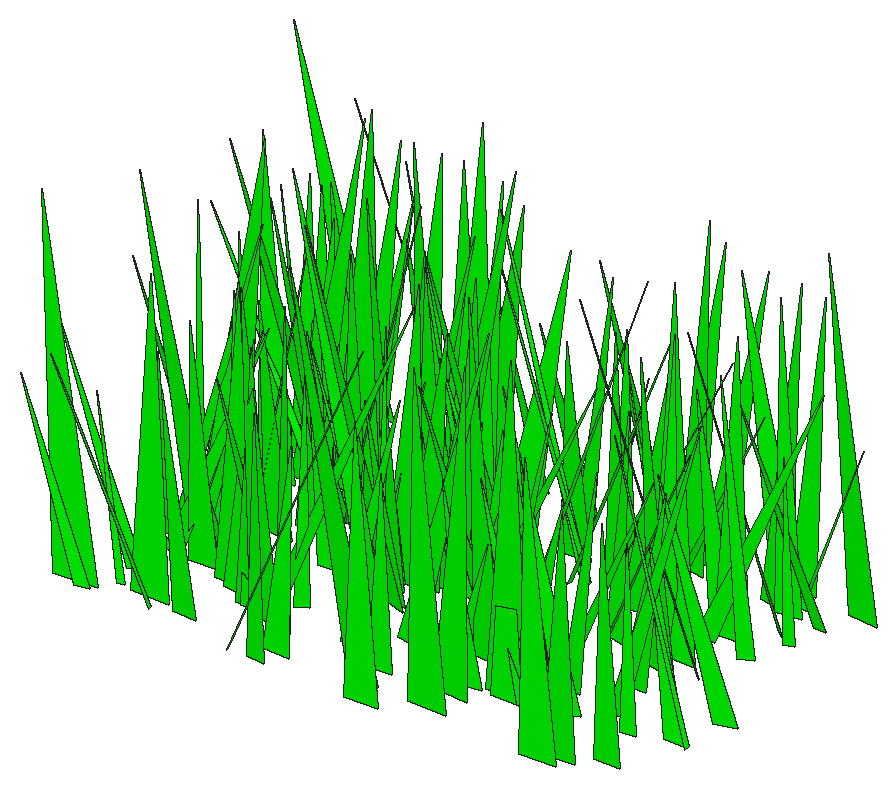
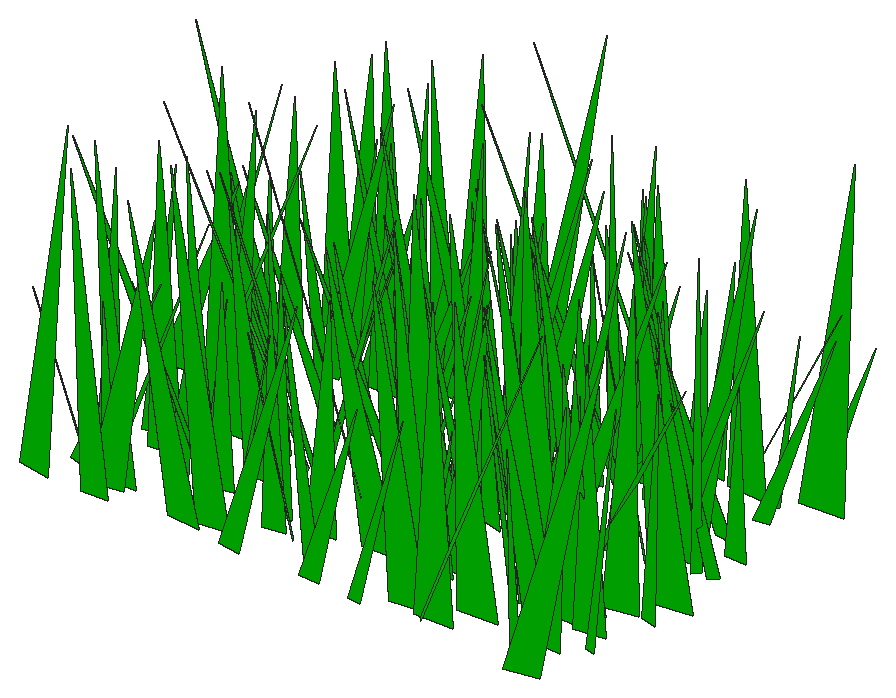
# SketchUp Ruby script. Lengths in inches.
U = 1.inch
M = Sketchup.active_model
def pt(a) = Geom::Point3d.new(a.map { |v| v * U })
def face(e, loops, mat)
  f = e.add_face(loops[0].map { |a| pt(a) })
  loops[1..].each { |l| e.add_face(l.map { |a| pt(a) }).erase! }
  f.material = f.back_material = mat if mat
  f
end
# faces: each face lists its corners as indices into pts; further lists are holes
def faces(e, pts, list, mat = nil) = list.each { |f| face(e, (f[0].is_a?(Array) ? f : [f]).map { |l| l.map { |i| pts[i] } }, mat) }
# xy, xz, yz: faces in a plane at the given z, y or x. An outline is a flat list of corners, or four numbers for a rectangle; further outlines are holes
def ring(l) = l.size == 4 ? [[l[0], l[1]], [l[2], l[1]], [l[2], l[3]], [l[0], l[3]]] : l.each_slice(2).to_a
def flat(e, list, mat, &to3) = list.each { |f| face(e, (f[0].is_a?(Array) ? f : [f]).map { |l| ring(l).map { |u, v| to3.(u, v) } }, mat) }
def xy(e, z, list, mat = nil) = flat(e, list, mat) { |x, y| [x, y, z] }
def xz(e, y, list, mat = nil) = flat(e, list, mat) { |x, z| [x, y, z] }
def yz(e, x, list, mat = nil) = flat(e, list, mat) { |y, z| [x, y, z] }
def lines(e, pts, list) = list.each { |a, b| e.add_line(pt(pts[a]), pt(pts[b])) }
# prism: a flat outline (further loops are holes) pulled along v
def prism(e, loops, v, mat = nil)
  f = face(e, loops, mat); d = Geom::Vector3d.new(v.map { |x| x * U })
  f.pushpull(f.normal.samedirection?(d) ? d.length : -d.length)
end
def box(e, o, s, mat = nil) = prism(e, [[o, [o[0] + s[0], o[1], o[2]], [o[0] + s[0], o[1] + s[1], o[2]], [o[0], o[1] + s[1], o[2]]]], [0, 0, s[2]], mat)
def at(x, y, z, deg = 0) = Geom::Transformation.translation(pt([x, y, z])) * Geom::Transformation.rotation(ORIGIN, Z_AXIS, deg.degrees)
def axes(o, x, y, z) = Geom::Transformation.new([*x, 0, *y, 0, *z, 0, *pt(o).to_a, 1])
def part(name) = M.definitions.add(name)
# library, detail: a bought-in or finely detailed component or shape, given as its bounding box
def library(name, o, s) = part(name).tap { |d| box(d.entities, o, s) }
def detail(e, o, s) = box(e.add_group.entities, o, s)
def put(e, d, t, mat = nil) = e.add_instance(d, t).tap { |i| i.material = mat if mat }
def group(e, t, mat = nil) = e.add_group.tap { |g| g.transformation = t; g.material = mat if mat }.entities
root = M.entities
M.materials.add("[0065_Lime]").color = [0, 255, 0]
c1 = part("fur_instance\#9")
p = [[0.8125,0,1.79],[0.67,-0.02,1.48],[0,-0.11,0],[0,0.11,0]]
faces(c1.entities,p,[[0,1,2,3]])
put(root,c1,axes([8.9,33.35,1.48],[-6.0138,0.86175,0.63827],[-6.15239,-0.84931,0.07042],[0.61144,-0.07017,6.98628]),"[0065_Lime]")
put(root,c1,axes([8.46,18.86,1.48],[-3.88652,0.33545,0.18947],[-2.38661,-0.54705,0.06343],[0.23932,-0.00778,3.70955]),"[0065_Lime]")
put(root,c1,axes([8.04,19.07,1.48],[-3.36903,1.09737,1.44562],[-7.991,-0.47878,-0.1432],[0.5387,-0.23927,6.91674]),"[0065_Lime]")
put(root,c1,axes([9.07,20.82,1.48],[-4.50342,0.37086,0.3157],[-2.65623,-0.63328,-0.14196],[0.24618,-0.04878,4.24348]),"[0065_Lime]")
put(root,c1,axes([7.81,28.21,1.48],[-4.12314,-0.37427,1.71758],[2.98502,-0.62181,0.2008],[1.62561,0.19252,3.98768]),"[0065_Lime]")
put(root,c1,axes([8.11,30.82,1.48],[-5.01442,-0.3098,1.44437],[2.22393,-0.74514,-0.2471],[1.75154,0.05919,4.44877]),"[0065_Lime]")
put(root,c1,axes([8.18,23.28,1.48],[-1.14454,-0.47717,1.57277],[3.88624,-0.16861,0.15702],[0.4088,0.26694,2.91062]),"[0065_Lime]")
put(root,c1,axes([10.8125,28.22,1.48],[-6.11625,0.18034,0.08013],[-1.2786,-0.85896,0.2057],[0.14827,0.03194,5.07922]),"[0065_Lime]")
put(root,c1,axes([8.93,28.23,1.48],[-4.40961,0.85616,1.82135],[-6.30115,-0.65595,0.23862],[1.55976,-0.22948,6.11318]),"[0065_Lime]")
put(root,c1,axes([8.6,24.73,1.48],[-6.54034,0.16656,2.37958],[-1.22942,-1.00551,0.12271],[2.90719,-0.0505,5.40528]),"[0065_Lime]")
put(root,c1,axes([10.26,23.64,1.48],[-5.48335,-0.42472,0.6271],[3.05756,-0.7752,0.09624],[0.6175,0.06696,5.09204]),"[0065_Lime]")
put(root,c1,axes([9.94,23.29,1.48],[-5.93025,-0.75535,1.74824],[5.64398,-0.85057,0.35258],[1.28866,0.24926,6.50099]),"[0065_Lime]")
put(root,c1,axes([8.82,29.96,1.48],[-2.26807,0.83828,1.07767],[-6.04515,-0.33684,0.36198],[0.89451,-0.1509,5.17876]),"[0065_Lime]")
put(root,c1,axes([7.77,27.07,1.48],[3.47067,-1.05454,1.7066],[7.77534,0.49003,-0.31581],[-0.51613,0.29092,6.71818]),"[0065_Lime]")
put(root,c1,axes([9.32,19.79,1.48],[-3.89594,0.16196,0.9526],[-1.14686,-0.57128,0.15127],[1.17673,-0.02056,3.30132]),"[0065_Lime]")
put(root,c1,axes([9.41,31.51,1.48],[-1.14326,0.75941,1.42467],[-5.68096,-0.15122,-0.31534],[-0.03629,-0.25202,4.48218]),"[0065_Lime]")
put(root,c1,axes([11.02,19.15,1.48],[-5.33918,-0.02324,0.11681],[0.17213,-0.74964,0.2073],[0.13548,0.03643,4.34009]),"[0065_Lime]")
put(root,c1,axes([9.51,29.79,1.48],[-0.06848,0.93849,0.05433],[-6.67345,-0.00923,-0.22485],[-0.27574,-0.00978,5.42826]),"[0065_Lime]")
put(root,c1,axes([9.3,33.17,1.48],[4.01234,0.3475,1.42745],[-2.5054,0.6103,-0.31901],[-1.70832,-0.07888,3.82051]),"[0065_Lime]")
put(root,c1,axes([7.98,24.67,1.48],[7.25075,-0.21832,1.21478],[1.60505,1.0386,-0.08405],[-1.43806,0.05845,6.03115]),"[0065_Lime]")
put(root,c1,axes([9.4,24.34,1.48],[1.30446,0.82547,0.45858],[-5.89734,0.18538,-0.08232],[-0.22142,-0.07423,4.89409]),"[0065_Lime]")
put(root,c1,axes([9.625,29.45,1.48],[-1.21215,0.77936,1.31455],[-5.71927,-0.19461,0.37691],[0.81457,-0.20666,4.60254]),"[0065_Lime]")
put(root,c1,axes([12.14,27.43,1.48],[-6.54248,-0.70335,0.85475],[5.07502,-0.92252,0.26449],[0.63475,0.12624,6.69537]),"[0065_Lime]")
put(root,c1,axes([10.6,22.42,1.48],[-0.37061,-0.71782,1.66325],[5.50113,-0.04198,0.2039],[-0.12143,0.28898,4.16119]),"[0065_Lime]")
put(root,c1,axes([10.46,24.35,1.48],[-3.94678,0.47191,1.9956],[-3.78114,-0.60508,-0.15314],[1.73225,-0.24556,4.21253]),"[0065_Lime]")
put(root,c1,axes([10.59,19.68,1.48],[1.30498,0.97324,1.79044],[-7.23587,0.20327,-0.21294],[-0.6768,-0.29661,5.72895]),"[0065_Lime]")
put(root,c1,axes([10.91,28.12,1.48],[-3.41033,-0.33839,1.42308],[2.61205,-0.51949,0.00234],[1.42733,0.14216,3.3959]),"[0065_Lime]")
put(root,c1,axes([9.81,28.71,1.48],[5.71666,0.90772,1.58932],[-6.58842,0.8286,-0.17845],[-1.46291,-0.18459,7.01433]),"[0065_Lime]")
put(root,c1,axes([9.46,23.67,1.48],[5.37143,-0.24513,0.64503],[1.69884,0.76259,0.35077],[-0.88652,-0.02388,4.58042]),"[0065_Lime]")
put(root,c1,axes([11.3,25.39,1.48],[-1.74942,-0.71538,0.93678],[5.19633,-0.25482,-0.10017],[0.49327,0.14726,4.37765]),"[0065_Lime]")
put(root,c1,axes([9.31,22.43,1.48],[5.08039,0.51052,0.33218],[-3.64812,0.71434,0.12789],[-0.24042,-0.05138,5.07881]),"[0065_Lime]")
put(root,c1,axes([13.73,32.5,1.48],[-7.84339,-0.14287,0.6675],[1.04981,-1.10687,0.22309],[0.77787,0.05324,6.42943]),"[0065_Lime]")
put(root,c1,axes([10.54,31.52,1.48],[5.82844,-0.08598,1.49258],[0.55601,0.85853,0.22057],[-1.85265,-0.01282,4.76187]),"[0065_Lime]")
put(root,c1,axes([10.45,25.09,1.48],[6.52819,0.11704,1.42515],[-0.79553,0.94978,-0.20267],[-1.76936,0.0048,5.34932]),"[0065_Lime]")
put(root,c1,axes([10.56,30.52,1.48],[5.59188,-0.51565,1.16817],[3.74043,0.80479,0.05725],[-1.24011,0.10226,5.44017]),"[0065_Lime]")
put(root,c1,axes([12.2,19.42,1.48],[-2.27237,-0.59666,1.29131],[4.4958,-0.32861,0.14666],[0.58115,0.20913,3.91462]),"[0065_Lime]")
put(root,c1,axes([11.46,27.26,1.48],[1.78465,0.48869,0.92062],[-3.6343,0.25678,0.09386],[-0.40963,-0.14914,3.17821]),"[0065_Lime]")
put(root,c1,axes([11.59,29.04,1.48],[-0.00433,-1.1966,2.59802],[9.08522,-0.02134,-0.31936],[0.42095,0.4483,6.91941]),"[0065_Lime]")
put(root,c1,axes([13.26,25.95,1.48],[-6.27713,-0.61141,1.23692],[4.3651,-0.90449,-0.32483],[1.48002,0.07454,6.20411]),"[0065_Lime]")
put(root,c1,axes([11.94,26.27,1.48],[-0.75546,0.72558,2.22199],[-5.81757,-0.12857,0.0981],[0.53004,-0.37694,4.24373]),"[0065_Lime]")
put(root,c1,axes([11.18,29.7,1.48],[5.74624,-0.80045,1.87909],[5.94432,0.83676,-0.08321],[-1.56558,0.23913,6.58102]),"[0065_Lime]")
put(root,c1,axes([12.23,28.12,1.48],[3.19662,0.59227,2.18587],[-4.77097,0.49525,0.11973],[-1.49168,-0.31477,4.30129]),"[0065_Lime]")
put(root,c1,axes([12.29,31.35,1.48],[0.0199,1.05878,0.85678],[-7.60428,-0.00195,0.19764],[0.24255,-0.14802,6.12581]),"[0065_Lime]")
put(root,c1,axes([12.21,21.97,1.48],[0.00108,-1.02135,0.84775],[7.33336,-0.00729,-0.3006],[0.37318,0.14627,5.90466]),"[0065_Lime]")
put(root,c1,axes([12.57,21.66,1.48],[-2.43132,-0.64779,2.29378],[5.20447,-0.39768,-0.11339],[1.45521,0.33998,4.23787]),"[0065_Lime]")
put(root,c1,axes([14.1875,26.22,1.48],[-4.24652,0.11497,0.68365],[-0.91798,-0.60188,-0.3811],[0.73013,-0.08807,3.497]),"[0065_Lime]")
put(root,c1,axes([14.2,21.59,1.48],[-3.58105,-0.50386,0.54129],[3.62286,-0.50653,0.05864],[0.41875,0.07338,4.12172]),"[0065_Lime]")
put(root,c1,axes([13.24,32.4375,1.48],[1.68019,-0.93968,1.82913],[7.02543,0.25267,0.07986],[-0.64806,0.30289,5.60803]),"[0065_Lime]")
put(root,c1,axes([14,24.74,1.48],[-1.63112,0.69601,0.67512],[-5.02222,-0.22632,-0.20976],[0.01127,-0.12212,4.23662]),"[0065_Lime]")
put(root,c1,axes([15.19,25.36,1.48],[-6.90925,0.71806,1.1047],[-5.16517,-0.98375,0.05269],[1.13087,-0.10607,6.99]),"[0065_Lime]")
put(root,c1,axes([13.54,21.16,1.48],[-2.16992,0.41998,1.45633],[-3.35484,-0.33184,-0.10058],[0.94007,-0.21482,3.00263]),"[0065_Lime]")
put(root,c1,axes([13.63,21.23,1.48],[1.53366,-0.93771,0.10175],[6.66075,0.21618,0.33288],[-0.42688,0.00422,5.55965]),"[0065_Lime]")
put(root,c1,axes([14.42,20.78,1.48],[-4.37564,-0.81327,1.84947],[6.02048,-0.65182,-0.18029],[1.55586,0.23506,5.89902]),"[0065_Lime]")
put(root,c1,axes([12.5,27.22,1.48],[7.91069,0.07287,1.50514],[-0.52519,1.14153,-0.0256],[-1.84854,-0.01248,6.44842]),"[0065_Lime]")
put(root,c1,axes([14.87,29.52,1.48],[-3.00734,-0.81287,0.74128],[5.8162,-0.43137,-0.23865],[0.68278,0.0943,5.29793]),"[0065_Lime]")
put(root,c1,axes([15.74,29.62,1.48],[-7.65414,0.04434,1.59511],[-0.22376,-1.10932,0.32293],[1.97359,0.0462,6.2229]),"[0065_Lime]")
put(root,c1,axes([13.49,29.68,1.48],[5.60131,0.48372,1.26107],[-3.56131,0.80635,0.10183],[-1.25326,-0.12944,5.34685]),"[0065_Lime]")
put(root,c1,axes([14.78,22.22,1.48],[4.48858,-0.34306,1.54729],[2.44196,0.68185,0.37878],[-1.9015,0.06585,4.1389]),"[0065_Lime]")
put(root,c1,axes([16.05,33,1.48],[-3.77265,-0.36392,0.57789],[2.59424,-0.53836,-0.15506],[0.69439,0.0341,3.719]),"[0065_Lime]")
put(root,c1,axes([15.21,20.71,1.48],[5.98257,0.4457,2.52464],[-3.57356,0.91789,0.1729],[-2.6313,-0.23322,5.50523]),"[0065_Lime]")
put(root,c1,axes([14.45,32.23,1.48],[1.84056,-0.97227,0.84239],[6.9937,0.25161,-0.3794],[0.18979,0.15736,5.81152]),"[0065_Lime]")
put(root,c1,axes([17.0625,24.09,1.48],[-7.17626,-0.57779,1.13591],[4.11781,-1.02577,-0.27127],[1.37883,0.05624,6.7221]),"[0065_Lime]")
put(root,c1,axes([15.45,29.98,1.48],[-0.45815,1.30829,0.76562],[-9.35691,-0.06602,0.07569],[0.13968,-0.13145,7.58207]),"[0065_Lime]")
put(root,c1,axes([15.8,27.68,1.48],[-5.36276,-0.94405,2.77604],[7.25656,-0.80564,0.09446],[2.03125,0.38572,6.99167]),"[0065_Lime]")
put(root,c1,axes([15.15,30.79,1.48],[5.56786,-0.67247,2.13279],[5.11241,0.82689,-0.09421],[-1.90805,0.25324,5.97125]),"[0065_Lime]")
put(root,c1,axes([15.78,18.6,1.48],[3.81296,0.48728,1.78687],[-3.6906,0.59139,-0.19341],[-1.79734,-0.1806,4.18788]),"[0065_Lime]")
put(root,c1,axes([16.28,25.1,1.48],[-7.12718,-0.57473,2.4408],[4.32401,-1.06852,-0.07697],[2.65255,0.19758,6.6837]),"[0065_Lime]")
put(root,c1,axes([15.85,25.48,1.48],[-1.04341,-0.732,0.20593],[5.19346,-0.14915,-0.35522],[0.47824,0.0227,4.30684]),"[0065_Lime]")
put(root,c1,axes([17.47,29.11,1.48],[-5.15823,-0.51821,0.78869],[3.74798,-0.73122,0.11928],[0.70227,0.09618,5.15644]),"[0065_Lime]")
put(root,c1,axes([15.6875,26.43,1.48],[-5.38941,-0.49484,2.8448],[4.08796,-0.85398,0.14654],[2.81447,0.29283,5.23464]),"[0065_Lime]")
put(root,c1,axes([16.03,24.68,1.48],[-5.40166,0.1449,2.12556],[-1.11266,-0.84109,0.05045],[2.5795,-0.05937,4.47284]),"[0065_Lime]")
put(root,c1,axes([17.44,28.77,1.48],[-3.92259,0.17784,0.34336],[-1.25087,-0.5543,0.16507],[0.46388,0.00909,3.34858]),"[0065_Lime]")
put(root,c1,axes([16.02,19.35,1.48],[-1.56349,0.605,1.29843],[-4.48418,-0.25218,0.36485],[0.98871,-0.18704,3.70801]),"[0065_Lime]")
put(root,c1,axes([15.46,25.46,1.48],[4.63251,-0.22591,0.81644],[1.58956,0.66595,0.20728],[-1.03223,0.01165,3.98323]),"[0065_Lime]")
put(root,c1,axes([16.9375,24.34,1.48],[-2.78367,-0.53198,0.51669],[3.77119,-0.39957,-0.3425],[0.7171,0.03625,3.80693]),"[0065_Lime]")
put(root,c1,axes([13.93,22.03,1.48],[7.67893,0.48609,0.31661],[-3.44023,1.07991,-0.35144],[-0.53208,0.03298,6.84167]),"[0065_Lime]")
put(root,c1,axes([16.33,25.5,1.48],[0.60845,-1.02133,1.0993],[7.38706,0.07639,-0.32697],[0.29482,0.19375,5.92384]),"[0065_Lime]")
put(root,c1,axes([17.6,25.99,1.48],[-3.08917,-0.49683,0.88059],[3.62946,-0.44531,0.00526],[0.7073,0.11517,3.81908]),"[0065_Lime]")
put(root,c1,axes([15.86,28.2,1.48],[-5.84392,-0.6732,4.36328],[5.88389,-1.00603,0.01288],[4.13601,0.47999,6.14672]),"[0065_Lime]")
put(root,c1,axes([18.0625,32.77,1.48],[-2.18033,-0.55083,0.03915],[3.91898,-0.30645,-0.07213],[0.10088,-0.00015,3.64789]),"[0065_Lime]")
put(root,c1,axes([16.22,22.79,1.48],[4.71105,-0.37176,0.96325],[2.75121,0.67347,-0.19307],[-0.91255,0.11117,4.39071]),"[0065_Lime]")
put(root,c1,axes([14.58,18.7,1.48],[8.4362,0.06423,0.60747],[-0.47416,1.18969,0.14194],[-0.73609,-0.03026,6.87071]),"[0065_Lime]")
put(root,c1,axes([16.88,25.71,1.48],[1.08644,-0.90471,0.57343],[6.46854,0.14645,-0.36608],[0.32933,0.10803,5.29852]),"[0065_Lime]")
put(root,c1,axes([17.37,21.35,1.48],[3.4959,-0.30181,1.17883],[2.2999,0.51896,-0.06044],[-1.19335,0.11602,3.33689]),"[0065_Lime]")
put(root,c1,axes([17.28,27.42,1.48],[0.4854,-1.03035,0.70236],[7.37596,0.06228,-0.31104],[0.32722,0.12448,5.96935]),"[0065_Lime]")
put(root,c1,axes([19.23,19.76,1.48],[-6.43107,-0.92142,1.38862],[6.61204,-0.92567,-0.32152],[1.48127,0.13155,7.46398]),"[0065_Lime]")
put(root,c1,axes([17.36,30.01,1.48],[1.57388,0.9876,0.51191],[-7.05243,0.21711,0.31085],[0.23701,-0.09795,5.85024]),"[0065_Lime]")
put(root,c1,axes([18.98,20.99,1.48],[-1.47595,-0.6345,1.08842],[4.70713,-0.20505,0.21784],[0.15061,0.19058,3.85801]),"[0065_Lime]")
put(root,c1,axes([20.45,29.55,1.48],[-7.60093,0.09893,1.26127],[-0.70463,-1.09001,0.05525],[1.55032,-0.0104,6.20892]),"[0065_Lime]")
put(root,c1,axes([18.57,26,1.48],[3.79111,-0.10032,1.23153],[0.87143,0.56799,-0.22453],[-1.42918,0.08022,3.1299]),"[0065_Lime]")
put(root,c1,axes([18.51,32.07,1.48],[4.56968,0.47129,1.36389],[-3.43179,0.67532,-0.21188],[-1.51103,-0.10849,4.60589]),"[0065_Lime]")
put(root,c1,axes([21.05,29.11,1.48],[-6.79557,-0.0071,0.85503],[0.03378,-0.96614,-0.09119],[1.05184,-0.01484,5.527]),"[0065_Lime]")
put(root,c1,axes([19.32,20.54,1.48],[-1.58465,0.52806,1.6693],[-4.21167,-0.24766,-0.02004],[0.77195,-0.26722,3.31739]),"[0065_Lime]")
put(root,c1,axes([19.6,30.24,1.48],[0.352,-0.79168,0.02398],[5.63357,0.04951,0.06076],[-0.0764,0.00348,4.59131]),"[0065_Lime]")
put(root,c1,axes([21.08,24.19,1.48],[-4.25349,-0.52668,0.42854],[3.76744,-0.59984,0.03789],[0.36433,0.05387,4.61133]),"[0065_Lime]")
put(root,c1,axes([20.16,18.52,1.48],[0.09562,0.90086,0.63467],[-6.4446,0.02045,-0.33042],[-0.42078,-0.10855,5.20491]),"[0065_Lime]")
put(root,c1,axes([19.67,25.57,1.48],[0.50546,0.59207,0.72695],[-4.30719,0.06879,0.10423],[0.02362,-0.12682,3.45033]),"[0065_Lime]")
put(root,c1,axes([21.32,32.8,1.48],[-4.48029,-0.5955,0.76956],[4.29776,-0.6354,0.07922],[0.61953,0.1014,5.01574]),"[0065_Lime]")
put(root,c1,axes([18.96,22.53,1.48],[5.99945,0.69589,1.18755],[-5.05495,0.85571,0.0939],[-1.05102,-0.14331,6.32717]),"[0065_Lime]")
put(root,c1,axes([20.08,31.08,1.48],[4.32609,0.07517,0.77088],[-0.5529,0.62199,0.0205],[-0.93736,-0.01994,3.54564]),"[0065_Lime]")
put(root,c1,axes([18.87,26.95,1.48],[5.7521,-0.21743,0.28749],[1.57094,0.80656,-0.35613],[-0.22645,0.07238,4.83206]),"[0065_Lime]")
put(root,c1,axes([20.92,30.99,1.48],[3.24773,-0.52797,1.65117],[4.05039,0.4944,0.02609],[-1.35364,0.21261,4.03965]),"[0065_Lime]")
put(root,c1,axes([21.61,23.18,1.48],[-5.53213,-0.70663,2.64819],[5.61999,-0.82781,0.3661],[2.07451,0.3582,6.07018]),"[0065_Lime]")
put(root,c1,axes([21.36,30.07,1.48],[-3.32584,-0.52363,2.00032],[4.20779,-0.51168,0.14054],[1.49281,0.27568,4.06037]),"[0065_Lime]")
put(root,c1,axes([22.24,21.5,1.48],[-0.9779,0.62717,0.1425],[-4.45105,-0.13471,-0.34233],[-0.37407,-0.03661,3.70083]),"[0065_Lime]")
put(root,c1,axes([20.56,23.3,1.48],[3.88025,-0.39387,0.59857],[2.84489,0.55064,-0.06068],[-0.55224,0.06914,3.89315]),"[0065_Lime]")
put(root,c1,axes([22.33,31.15,1.48],[-4.37535,0.05439,1],[-0.42453,-0.63805,-0.06604],[1.21696,-0.02702,3.57226]),"[0065_Lime]")
put(root,c1,axes([22.05,19.5625,1.48],[-2.13137,-0.93201,2.63311],[7.3518,-0.30981,0.2628],[0.6501,0.44791,5.66074]),"[0065_Lime]")
put(root,c1,axes([19.98,27.67,1.48],[8.26328,0.17029,0.99565],[-1.24964,1.17277,0.14051],[-1.1855,-0.04923,6.79191]),"[0065_Lime]")
put(root,c1,axes([22.1,20.68,1.48],[3.62413,0.86524,2.18094],[-6.57617,0.54409,-0.00285],[-1.36322,-0.32443,5.81176]),"[0065_Lime]")
put(root,c1,axes([20.49,28.8125,1.48],[7.08757,-0.00562,0.63888],[0.06455,1.00153,-0.17849],[-0.7838,0.03165,5.76245]),"[0065_Lime]")
put(root,c1,axes([22.5,24.18,1.48],[2.2355,-0.49086,0.30339],[3.51204,0.31378,-0.11074],[-0.08581,0.05447,3.37165]),"[0065_Lime]")
put(root,c1,axes([22.97,31.82,1.48],[-5.18025,-0.72118,3.06538],[5.70879,-0.82839,-0.14746],[2.81992,0.35222,5.92969]),"[0065_Lime]")
put(root,c1,axes([24.5625,21.56,1.48],[-3.34419,0.51735,0.35719],[-3.69551,-0.47183,0.00748],[0.30208,-0.0448,4.04576]),"[0065_Lime]")
put(root,c1,axes([22.57,32.09,1.48],[5.49021,-0.74763,1.72421],[5.53997,0.79791,-0.07813],[-1.45272,0.21733,6.21831]),"[0065_Lime]")
put(root,c1,axes([23.7,21.55,1.48],[-0.98731,0.78716,1.21784],[-5.7899,-0.14546,0.04482],[0.31598,-0.20579,4.62666]),"[0065_Lime]")
put(root,c1,axes([23.89,29.96,1.48],[-2.19586,0.61762,0.86702],[-4.44172,-0.32587,0.33542],[0.85216,-0.10702,3.98246]),"[0065_Lime]")
put(root,c1,axes([23.57,21.74,1.48],[1.86184,-1.05066,1.75181],[7.75717,0.275,0.07196],[-0.60948,0.29052,6.26727]),"[0065_Lime]")
put(root,c1,axes([22.91,21.84,1.48],[5.99179,0.43053,1.22519],[-3.08122,0.86604,-0.22755],[-1.47043,-0.06041,5.46929]),"[0065_Lime]")
put(root,c1,axes([23.31,28.7,1.48],[3.43306,-0.74352,0.25578],[5.27112,0.48442,0.3758],[-0.55875,0.00159,5.11678]),"[0065_Lime]")
put(root,c1,axes([23.92,26.81,1.48],[3.61143,0.48651,1.56528],[-3.73303,0.5404,0.07038],[-1.32473,-0.19651,4.06888]),"[0065_Lime]")
put(root,c1,axes([24.76,29.79,1.48],[-3.94473,-0.16794,1.06228],[1.19285,-0.58333,-0.15952],[1.30808,0.02549,3.34894]),"[0065_Lime]")
put(root,c1,axes([23.51,32.4,1.48],[3.89702,0.87086,0.86418],[-6.24618,0.55635,-0.15013],[-0.72324,-0.11239,5.95304]),"[0065_Lime]")
put(root,c1,axes([25.89,22.05,1.48],[-6.03856,0.46302,1.24581],[-3.44339,-0.86247,-0.30181],[1.1604,-0.14983,5.5874]),"[0065_Lime]")
put(root,c1,axes([25.22,21.75,1.48],[4.28873,0.35496,2.33104],[-2.84544,0.70078,-0.11199],[-2.54894,-0.18506,4.04711]),"[0065_Lime]")
put(root,c1,axes([25.48,30.35,1.48],[-1.95158,0.63014,0.50398],[-4.52447,-0.27467,-0.08417],[0.15154,-0.08566,3.97723]),"[0065_Lime]")
put(root,c1,axes([23.1,31.22,1.48],[4.77313,-0.1232,0.15482],[0.87714,0.67123,0.00567],[-0.18846,0.00387,3.94747]),"[0065_Lime]")
put(root,c1,axes([27.54,26.56,1.48],[-7.89203,-0.15983,0.75748],[1.15423,-1.11627,0.06401],[0.91037,0.02969,6.4855]),"[0065_Lime]")
put(root,c1,axes([24.89,23.38,1.48],[3.55784,0.48501,1.31828],[-3.66087,0.52161,0.10659],[-1.06683,-0.17242,4.03067]),"[0065_Lime]")
put(root,c1,axes([22.51,27.27,1.48],[7.77015,0.06985,0.19767],[-0.50028,1.09227,0.07814],[-0.23636,-0.01566,6.33278]),"[0065_Lime]")
put(root,c1,axes([26.92,32.12,1.48],[-4.09581,0.89049,0.05554],[-6.32539,-0.5751,0.34419],[0.3924,0.02423,6.128]),"[0065_Lime]")
put(root,c1,axes([23.87,24.5,1.48],[5.18477,-0.24235,0.21914],[1.71999,0.72951,0.10951],[-0.29811,-0.00603,4.44323]),"[0065_Lime]")
put(root,c1,axes([27.85,30.41,1.48],[-6.26726,-0.16099,0.62956],[1.14967,-0.88723,-0.03001],[0.76802,0.01442,5.18226]),"[0065_Lime]")
put(root,c1,axes([24.2,25.74,1.48],[5.62947,0.03791,0.43337],[-0.24011,0.79347,-0.26223],[-0.5468,0.04187,4.57684]),"[0065_Lime]")
put(root,c1,axes([25.86,26.97,1.48],[5.86427,-0.49194,2.42229],[3.88857,0.89267,-0.15384],[-2.4502,0.23931,5.55331]),"[0065_Lime]")
put(root,c1,axes([26.13,26.99,1.48],[-1.73027,1.12623,2.07371],[-8.38026,-0.26189,0.13954],[0.71347,-0.34476,6.66814]),"[0065_Lime]")
put(root,c1,axes([26.4375,26.08,1.48],[-4.55742,-0.7292,1.7323],[5.34511,-0.68149,-0.30859],[1.70149,0.1877,5.60936]),"[0065_Lime]")
put(root,c1,axes([26.93,19.11,1.48],[-0.29609,0.94167,1.06682],[-6.82002,-0.03154,-0.3194],[-0.34192,-0.18628,5.44701]),"[0065_Lime]")
put(root,c1,axes([26.85,29.15,1.48],[3.26001,-0.79586,2.15542],[6.11452,0.49362,-0.01149],[-1.30868,0.32378,5.31562]),"[0065_Lime]")
put(root,c1,axes([28.68,31.4,1.48],[-4.33813,-0.36524,0.28777],[2.62065,-0.60766,0.29521],[0.1157,0.06934,4.10299]),"[0065_Lime]")
put(root,c1,axes([27.29,31.53,1.48],[5.07124,-0.54785,2.67376],[4.43612,0.79522,-0.10707],[-2.51521,0.29795,5.20207]),"[0065_Lime]")
put(root,c1,axes([26.6,31.72,1.48],[-4.14323,-0.76486,2.83135],[5.96531,-0.67604,-0.34393],[2.48173,0.34807,5.55361]),"[0065_Lime]")
put(root,c1,axes([26.39,24.71,1.48],[2.60562,-0.58991,0.74926],[4.28468,0.36842,-0.13884],[-0.33794,0.12278,4.01667]),"[0065_Lime]")
put(root,c1,axes([27.01,31.84,1.48],[-2.13176,-0.44629,1.13769],[3.27087,-0.33546,-0.35443],[1.15963,0.12579,3.09114]),"[0065_Lime]")
put(root,c1,axes([26.82,32.81,1.48],[5.43477,-0.6209,1.5872],[4.48286,0.80205,0.35756],[-1.7989,0.12288,5.68622]),"[0065_Lime]")
put(root,c1,axes([28.04,28.41,1.48],[-5.37798,0.34953,1.84766],[-2.78863,-0.79927,-0.30385],[1.8896,-0.18475,4.81019]),"[0065_Lime]")
put(root,c1,axes([27.41,19.59,1.48],[1.76399,-0.84202,0.44268],[5.9988,0.25229,0.26469],[-0.46682,0.0603,5.0741]),"[0065_Lime]")
put(root,c1,axes([28.13,22.25,1.48],[-3.20094,0.35124,1.20556],[-2.56381,-0.4872,0.25245],[1.36806,-0.09121,3.29384]),"[0065_Lime]")
put(root,c1,axes([26.12,28.72,1.48],[5.67503,0.57768,0.07173],[-4.11168,0.79747,0.0236],[-0.05439,-0.01057,5.70006]),"[0065_Lime]")
put(root,c1,axes([28.55,29.97,1.48],[-3.5585,0.23447,1.34575],[-1.81997,-0.54188,-0.0205],[1.4863,-0.10217,3.19688]),"[0065_Lime]")
put(root,c1,axes([27.26,32.28,1.48],[4.14212,0.11334,0.4221],[-0.79995,0.58659,-0.08392],[-0.52908,0.0004,3.43151]),"[0065_Lime]")
put(root,c1,axes([28.81,20.33,1.48],[1.56988,0.68245,1.49966],[-5.1154,0.25024,-0.27286],[-0.90521,-0.23056,4.14279]),"[0065_Lime]")
put(root,c1,axes([30.23,24.61,1.48],[-3.21218,0.6138,0.11113],[-4.3624,-0.44891,-0.34599],[-0.26209,-0.05084,4.39678]),"[0065_Lime]")
put(root,c1,axes([30.17,22.72,1.48],[-6.57811,0.01174,1.1116],[-0.12675,-0.94357,-0.16222],[1.36326,-0.03106,5.34869]),"[0065_Lime]")
put(root,c1,axes([29.39,32.69,1.48],[-5.52023,-0.7583,2.25609],[5.80176,-0.81392,0.22549],[1.77615,0.30187,6.27533]),"[0065_Lime]")
put(root,c1,axes([27.04,22.99,1.48],[7.11778,-0.31852,1.19505],[2.39087,1.01366,-0.3686],[-1.25718,0.12437,6.06502]),"[0065_Lime]")
put(root,c1,axes([29.67,22.74,1.48],[-2.29983,0.53232,0.18082],[-3.78374,-0.32446,0.16583],[0.28972,-0.01179,3.60103]),"[0065_Lime]")
